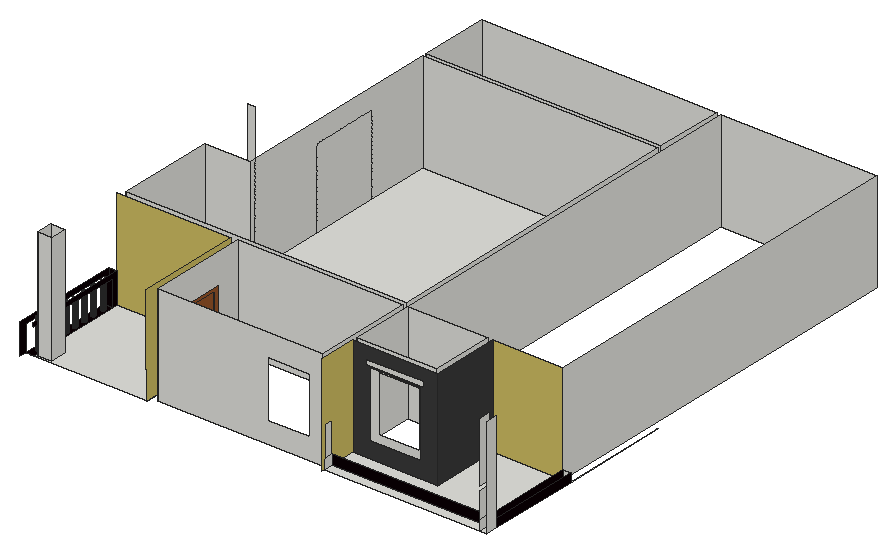
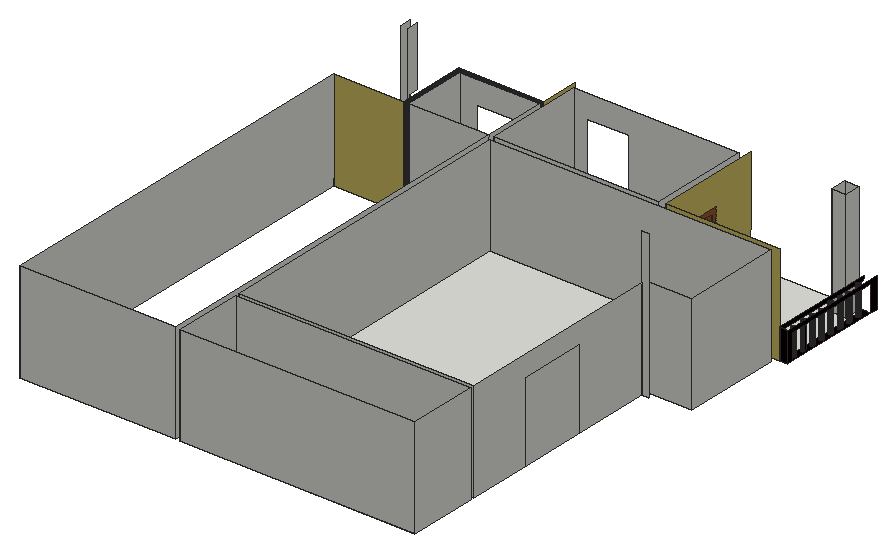
# SketchUp Ruby script. Lengths in inches.
U = 1.inch
M = Sketchup.active_model
def pt(a) = Geom::Point3d.new(a.map { |v| v * U })
def face(e, loops, mat)
  f = e.add_face(loops[0].map { |a| pt(a) })
  loops[1..].each { |l| e.add_face(l.map { |a| pt(a) }).erase! }
  f.material = f.back_material = mat if mat
  f
end
# faces: each face lists its corners as indices into pts; further lists are holes
def faces(e, pts, list, mat = nil) = list.each { |f| face(e, (f[0].is_a?(Array) ? f : [f]).map { |l| l.map { |i| pts[i] } }, mat) }
# xy, xz, yz: faces in a plane at the given z, y or x. An outline is a flat list of corners, or four numbers for a rectangle; further outlines are holes
def ring(l) = l.size == 4 ? [[l[0], l[1]], [l[2], l[1]], [l[2], l[3]], [l[0], l[3]]] : l.each_slice(2).to_a
def flat(e, list, mat, &to3) = list.each { |f| face(e, (f[0].is_a?(Array) ? f : [f]).map { |l| ring(l).map { |u, v| to3.(u, v) } }, mat) }
def xy(e, z, list, mat = nil) = flat(e, list, mat) { |x, y| [x, y, z] }
def xz(e, y, list, mat = nil) = flat(e, list, mat) { |x, z| [x, y, z] }
def yz(e, x, list, mat = nil) = flat(e, list, mat) { |y, z| [x, y, z] }
def lines(e, pts, list) = list.each { |a, b| e.add_line(pt(pts[a]), pt(pts[b])) }
# prism: a flat outline (further loops are holes) pulled along v
def prism(e, loops, v, mat = nil)
  f = face(e, loops, mat); d = Geom::Vector3d.new(v.map { |x| x * U })
  f.pushpull(f.normal.samedirection?(d) ? d.length : -d.length)
end
def box(e, o, s, mat = nil) = prism(e, [[o, [o[0] + s[0], o[1], o[2]], [o[0] + s[0], o[1] + s[1], o[2]], [o[0], o[1] + s[1], o[2]]]], [0, 0, s[2]], mat)
def at(x, y, z, deg = 0) = Geom::Transformation.translation(pt([x, y, z])) * Geom::Transformation.rotation(ORIGIN, Z_AXIS, deg.degrees)
def axes(o, x, y, z) = Geom::Transformation.new([*x, 0, *y, 0, *z, 0, *pt(o).to_a, 1])
def part(name) = M.definitions.add(name)
# library, detail: a bought-in or finely detailed component or shape, given as its bounding box
def library(name, o, s) = part(name).tap { |d| box(d.entities, o, s) }
def detail(e, o, s) = box(e.add_group.entities, o, s)
def put(e, d, t, mat = nil) = e.add_instance(d, t).tap { |i| i.material = mat if mat }
def group(e, t, mat = nil) = e.add_group.tap { |g| g.transformation = t; g.material = mat if mat }.entities
root = M.entities
M.materials.add("[Color D05]").color = [208, 191, 99]
M.materials.add("[Color E01]").color = [255, 255, 204]
M.materials.add("[Color M07]").color = [58, 58, 58]
M.materials.add("[Metal Seamed]").color = [11, 0, 4]
M.materials.add("[Wood Cherry Original]").color = [152, 86, 42]
c1 = part("Group\#1")
xy(c1.entities,0,[[0,0,6.3125,48]],"[Wood Cherry Original]")
xy(c1.entities,4.83,[[2.3125,4.83,3.9375,43.17]])
xy(c1.entities,4.83,[[0,4.83,2.3125,43.17],[3.9375,4.83,6.3125,43.17]],"[Wood Cherry Original]")
xy(c1.entities,79.17,[[2.3125,4.83,3.9375,43.17]])
xy(c1.entities,79.17,[[0,4.83,2.3125,43.17],[3.9375,4.83,6.3125,43.17]],"[Wood Cherry Original]")
xy(c1.entities,84,[[0,0,6.3125,48]],"[Wood Cherry Original]")
xz(c1.entities,0,[[0,0,6.3125,84]],"[Wood Cherry Original]")
xz(c1.entities,4.83,[[2.3125,4.83,3.9375,79.17]])
xz(c1.entities,4.83,[[0,4.83,2.3125,79.17],[3.9375,4.83,6.3125,79.17]],"[Wood Cherry Original]")
xz(c1.entities,43.17,[[2.3125,4.83,3.9375,79.17]])
xz(c1.entities,43.17,[[0,4.83,2.3125,79.17],[3.9375,4.83,6.3125,79.17]],"[Wood Cherry Original]")
xz(c1.entities,48,[[0,0,6.3125,84]],"[Wood Cherry Original]")
yz(c1.entities,0,[[[0,0,48,84],[4.83,4.83,43.17,79.17]]],"[Wood Cherry Original]")
yz(c1.entities,2.3125,[[7.68,9.76,40.37,11.76],[7.68,18.32,40.37,20.32],[7.68,27.01,40.37,29.01],[7.68,35.69,40.37,37.69],[7.68,44.38,40.37,46.38],
  [7.68,53.07,40.37,55.07],[7.68,61.76,40.37,63.76],[7.68,70.44,40.37,72.44]],"[Color E01]")
yz(c1.entities,2.3125,[[[4.83,4.83,43.17,79.17],[7.68,70.44,40.37,72.44],[7.68,61.76,40.37,63.76],[7.68,53.07,40.37,55.07],[7.68,44.38,40.37,46.38],[7.68,35.69,40.37,37.69],[7.68,27.01,40.37,29.01],[7.68,18.32,40.37,20.32],[7.68,9.76,40.37,11.76]]],"[Wood Cherry Original]")
yz(c1.entities,3.9375,[[4.83,4.83,43.17,79.17]],"[Wood Cherry Original]")
yz(c1.entities,6.3125,[[[0,0,48,84],[4.83,4.83,43.17,79.17]]],"[Wood Cherry Original]")
xy(root,288,[[[21.75,70.73,158,195.41],[24.07,73.08,41.19,92.83]],[369.3125,70.97,555.7,82.57],[555.7,70.97,564.5,84.18],[24.07,73.08,41.19,92.83],[16.88,80.51,16.29,80.625,15.75,80.89,15.29,81.28,14.95,81.78,14.75,82.35,14.7,82.95,14.82,83.55,15.08,84.09,15.47,84.55,15.97,84.89,16.54,85.09,17.14,85.13,17.74,85.02,18.28,84.76,18.74,84.36,19.08,83.86,19.28,83.29,19.32,82.69,19.21,82.1,18.95,81.55,18.55,81.1,18.05,80.76,17.49,80.56],
  [369.3125,82.57,555.7,82.57,555.7,84.18,555.3125,195.41,471.3125,195.41,471.3125,113.66,369.3125,113.66],[555.7,84.18,555.3125,195.41,564.5,195.41,564.5,84.18],[16.88,94.39,16.29,94.5,15.75,94.76,15.29,95.16,14.95,95.66,14.75,96.23,14.7,96.83,14.82,97.42,15.08,97.96,15.47,98.42,15.97,98.76,16.54,98.96,17.14,99.01,17.74,98.89,18.28,98.63,18.74,98.24,19.08,97.74,19.28,97.17,19.32,96.57,19.21,95.97,18.95,95.43,18.55,94.97,18.05,94.63,17.49,94.43],[16.88,108.26,16.29,108.375,15.75,108.64,15.29,109.03,14.95,109.53,14.75,110.1,14.7,110.7,14.82,111.3,15.08,111.84,15.47,112.3,15.97,112.64,16.54,112.84,17.14,112.88,17.74,112.77,18.28,112.51,18.74,112.11,19.08,111.61,19.28,111.04,19.32,110.44,19.21,109.85,18.95,109.3,18.55,108.85,18.05,108.51,17.49,108.31],[158,120.11,165.5625,168.11],
  [16.88,122.14,16.29,122.25,15.75,122.51,15.29,122.91,14.95,123.41,14.75,123.98,14.7,124.58,14.82,125.17,15.08,125.71,15.47,126.17,15.97,126.51,16.54,126.71,17.14,126.76,17.74,126.64,18.28,126.38,18.74,125.99,19.08,125.49,19.28,124.92,19.32,124.32,19.21,123.72,18.95,123.18,18.55,122.72,18.05,122.38,17.49,122.18],[16.88,136.01,16.29,136.125,15.75,136.39,15.29,136.78,14.95,137.28,14.75,137.85,14.7,138.45,14.82,139.05,15.08,139.59,15.47,140.05,15.97,140.39,16.54,140.59,17.14,140.63,17.74,140.52,18.28,140.26,18.74,139.86,19.08,139.36,19.28,138.79,19.32,138.19,19.21,137.6,18.95,137.05,18.55,136.6,18.05,136.26,17.49,136.06],[16.88,149.89,16.29,150,15.75,150.26,15.29,150.66,14.95,151.16,14.75,151.73,14.7,152.33,14.82,152.92,15.08,153.46,15.47,153.92,15.97,154.26,16.54,154.46,17.14,154.51,17.74,154.39,18.28,154.13,18.74,153.74,19.08,153.24,19.28,152.67,19.32,152.07,19.21,151.47,18.95,150.93,18.55,150.47,18.05,150.13,17.49,149.93],[16.88,163.76,16.29,163.875,15.75,164.14,15.29,164.53,14.95,165.03,14.75,165.6,14.7,166.2,14.82,166.8,15.08,167.34,15.47,167.8,15.97,168.14,16.54,168.34,17.14,168.38,17.74,168.27,18.28,168.01,18.74,167.61,19.08,167.11,19.28,166.54,19.32,165.94,19.21,165.35,18.95,164.8,18.55,164.35,18.05,164.01,17.49,163.81],[16.88,177.64,16.29,177.75,15.75,178.01,15.29,178.41,14.95,178.91,14.75,179.48,14.7,180.08,14.82,180.67,15.08,181.21,15.47,181.67,15.97,182.01,16.54,182.21,17.14,182.26,17.74,182.14,18.28,181.88,18.74,181.49,19.08,180.99,19.28,180.42,19.32,179.82,19.21,179.22,18.95,178.68,18.55,178.22,18.05,177.88,17.49,177.68],
  [11.6875,188.88,21.75,195.41],[564.3125,195.41,564.5,326.53],[26.75,201.41,363.3125,201.41,363.3125,578.04,81.6875,578.04,81.6875,320.85,26.75,320.85],[81.6875,582.91,363.3125,665.75]])
xy(root,288,[[[11.6875,71.13,16.3,71.13,16.54,71.21,17.14,71.26,17.74,71.14,17.77,71.13,21.75,71.13,21.75,188.88,11.6875,188.88],[16.88,163.76,16.29,163.875,15.75,164.14,15.29,164.53,14.95,165.03,14.75,165.6,14.7,166.2,14.82,166.8,15.08,167.34,15.47,167.8,15.97,168.14,16.54,168.34,17.14,168.38,17.74,168.27,18.28,168.01,18.74,167.61,19.08,167.11,19.28,166.54,19.32,165.94,19.21,165.35,18.95,164.8,18.55,164.35,18.05,164.01,17.49,163.81],[16.88,149.89,16.29,150,15.75,150.26,15.29,150.66,14.95,151.16,14.75,151.73,14.7,152.33,14.82,152.92,15.08,153.46,15.47,153.92,15.97,154.26,16.54,154.46,17.14,154.51,17.74,154.39,18.28,154.13,18.74,153.74,19.08,153.24,19.28,152.67,19.32,152.07,19.21,151.47,18.95,150.93,18.55,150.47,18.05,150.13,17.49,149.93],[16.88,136.01,16.29,136.125,15.75,136.39,15.29,136.78,14.95,137.28,14.75,137.85,14.7,138.45,14.82,139.05,15.08,139.59,15.47,140.05,15.97,140.39,16.54,140.59,17.14,140.63,17.74,140.52,18.28,140.26,18.74,139.86,19.08,139.36,19.28,138.79,19.32,138.19,19.21,137.6,18.95,137.05,18.55,136.6,18.05,136.26,17.49,136.06],[16.88,122.14,16.29,122.25,15.75,122.51,15.29,122.91,14.95,123.41,14.75,123.98,14.7,124.58,14.82,125.17,15.08,125.71,15.47,126.17,15.97,126.51,16.54,126.71,17.14,126.76,17.74,126.64,18.28,126.38,18.74,125.99,19.08,125.49,19.28,124.92,19.32,124.32,19.21,123.72,18.95,123.18,18.55,122.72,18.05,122.38,17.49,122.18],[16.88,108.26,16.29,108.375,15.75,108.64,15.29,109.03,14.95,109.53,14.75,110.1,14.7,110.7,14.82,111.3,15.08,111.84,15.47,112.3,15.97,112.64,16.54,112.84,17.14,112.88,17.74,112.77,18.28,112.51,18.74,112.11,19.08,111.61,19.28,111.04,19.32,110.44,19.21,109.85,18.95,109.3,18.55,108.85,18.05,108.51,17.49,108.31],[16.88,94.39,16.29,94.5,15.75,94.76,15.29,95.16,14.95,95.66,14.75,96.23,14.7,96.83,14.82,97.42,15.08,97.96,15.47,98.42,15.97,98.76,16.54,98.96,17.14,99.01,17.74,98.89,18.28,98.63,18.74,98.24,19.08,97.74,19.28,97.17,19.32,96.57,19.21,95.97,18.95,95.43,18.55,94.97,18.05,94.63,17.49,94.43],[16.88,80.51,16.29,80.625,15.75,80.89,15.29,81.28,14.95,81.78,14.75,82.35,14.7,82.95,14.82,83.55,15.08,84.09,15.47,84.55,15.97,84.89,16.54,85.09,17.14,85.13,17.74,85.02,18.28,84.76,18.74,84.36,19.08,83.86,19.28,83.29,19.32,82.69,19.21,82.1,18.95,81.55,18.55,81.1,18.05,80.76,17.49,80.56],[16.88,177.64,16.29,177.75,15.75,178.01,15.29,178.41,14.95,178.91,14.75,179.48,14.7,180.08,14.82,180.67,15.08,181.21,15.47,181.67,15.97,182.01,16.54,182.21,17.14,182.26,17.74,182.14,18.28,181.88,18.74,181.49,19.08,180.99,19.28,180.42,19.32,179.82,19.21,179.22,18.95,178.68,18.55,178.22,18.05,177.88,17.49,177.68]]],"[Metal Seamed]")
xz(root,73.08,[[24.07,288,41.19,420.5]])
xz(root,76.28,[[[165.5625,288,363.3125,408],[297.45,313.04,347.52,380.98]]])
xz(root,82.57,[[369.3125,288,555.7,300]],"[Metal Seamed]")
xz(root,84.18,[[555.7,288,564.5,298.1875]])
xz(root,92.83,[[24.07,288,41.19,420.5]])
xz(root,113.66,[[[369.3125,288,471.3125,408],[389.45,307.48,450.64,386.54],[384.5,386.56,384.5,393.87,454.38,393.87,454.38,386.56,450.58,386.56,450.58,386.84,390.89,386.84,390.89,386.56]]],"[Color M07]")
xz(root,119.66,[[[369.3125,288,465.3125,408],[395.02,313.04,445.08,380.98]]])
xz(root,120.11,[[158,288,165.5625,372]])
xz(root,168.11,[[158,288,165.5625,372]])
xz(root,188.88,[[11.6875,288,21.75,318.96]],"[Metal Seamed]")
xz(root,195.41,[[165.5625,288,363.3125,408],[369.3125,288,465.3125,408],[555.3125,288,564.3125,298.1875],[564.3125,288,564.5,298.1875]])
xz(root,195.41,[[21.75,288,158,408],[471.3125,288,555.3125,408]],"[Color D05]")
xz(root,195.41,[[11.6875,288,21.75,324]],"[Metal Seamed]")
xz(root,201.41,[[26.75,288,363.3125,408]])
xz(root,320.85,[[26.75,288,81.6875,408]])
xz(root,326.53,[[72.6875,288,81.6875,464.125]])
xz(root,578.04,[[81.6875,288,363.3125,408]])
xz(root,582.91,[[81.6875,288,363.3125,408]])
xz(root,664.97,[[369.3125,288,555.3125,408]])
xz(root,665.75,[[81.6875,288,363.3125,408]])
yz(root,11.6875,[[62.76,288,62.76,324,195.41,324,195.41,288,188.88,288,188.88,318.96,71.13,318.96,71.13,288]],"[Metal Seamed]")
yz(root,21.75,[[188.88,288,195.41,288,195.41,324,69.57,324,69.57,320.52,71.13,320.52,71.13,318.96,188.88,318.96]],"[Metal Seamed]")
yz(root,24.07,[[73.08,288,92.83,420.5]])
yz(root,26.75,[[201.41,288,320.85,408]])
yz(root,41.19,[[73.08,288,92.83,420.5]])
yz(root,81.6875,[[320.85,288,326.53,408],[326.53,288,419.61,288,419.61,383.34,501.8,383.34,501.8,288,578.04,288,578.04,408,326.53,408],[419.61,288,501.8,383.34],[582.91,288,665.75,408]])
yz(root,158,[[69.57,288,69.57,324,67.28,324,67.28,408,195.41,408,195.41,288,168.11,288,168.11,372,120.11,372,120.11,288]],"[Color D05]")
yz(root,165.5625,[[76.28,288,120.11,288,120.11,372,168.11,372,168.11,288,195.41,288,195.41,408,76.28,408]])
yz(root,363.3125,[[76.28,288,195.41,408],[201.41,288,578.04,408],[582.91,288,665.75,408]])
yz(root,369.3125,[[70.97,288,82.57,300],[119.66,288,195.41,408],[195.41,288,664.97,408]])
yz(root,369.3125,[[67.28,288,70.97,288,70.97,336,82.57,336,82.57,288,113.66,288,113.66,408,67.28,408]],"[Color D05]")
yz(root,465.3125,[[119.66,288,195.41,408]])
yz(root,471.3125,[[113.66,288,195.41,408]],"[Color M07]")
yz(root,555.3125,[[195.41,288,664.97,408]])
yz(root,555.7,[[70.97,288,82.57,300],[82.57,288,82.57,300,70.97,300,70.97,331.08,82.57,331.08,82.57,336,70.97,336,70.97,408,84.18,408,84.18,288]])
yz(root,564.5,[[70.97,288,84.18,408]])
yz(root,564.5,[[84.18,288,195.41,298.1875]],"[Metal Seamed]")
p = [[16.29,80.625,288],[16.88,80.51,288],[16.88,80.51,322.6875],[16.29,80.625,322.6875],[17.49,80.56,288],[17.49,80.56,322.6875],
  [15.75,80.89,288],[15.75,80.89,322.6875],[18.05,80.76,288],[18.05,80.76,322.6875],[18.55,81.1,288],[18.55,81.1,322.6875],
  [15.29,81.28,288],[15.29,81.28,322.6875],[18.95,81.55,288],[18.95,81.55,322.6875],[14.95,81.78,288],[14.95,81.78,322.6875],
  [19.21,82.1,288],[19.21,82.1,322.6875],[14.75,82.35,288],[14.75,82.35,322.6875],[19.32,82.69,288],[19.32,82.69,322.6875],
  [14.7,82.95,288],[14.7,82.95,322.6875],[19.28,83.29,288],[19.28,83.29,322.6875],[14.82,83.55,288],[14.82,83.55,322.6875],
  [19.08,83.86,288],[19.08,83.86,322.6875],[15.08,84.09,288],[15.08,84.09,322.6875],[18.74,84.36,288],[18.74,84.36,322.6875],
  [15.47,84.55,288],[15.47,84.55,322.6875],[555.3125,195.41,288],[555.7,84.18,288],[555.7,84.18,298.1875],[555.3125,195.41,298.1875],
  [18.28,84.76,288],[18.28,84.76,322.6875],[15.97,84.89,288],[15.97,84.89,322.6875],[17.74,85.02,288],[17.74,85.02,322.6875],
  [16.54,85.09,288],[16.54,85.09,322.6875],[17.14,85.13,288],[17.14,85.13,322.6875],[16.29,94.5,288],[16.88,94.39,288],
  [16.88,94.39,318.96],[16.29,94.5,318.96],[17.49,94.43,288],[17.49,94.43,318.96],[18.05,94.63,288],[18.05,94.63,318.96],
  [15.75,94.76,288],[15.75,94.76,318.96],[18.55,94.97,288],[18.55,94.97,318.96],[15.29,95.16,288],[15.29,95.16,318.96],
  [18.95,95.43,288],[18.95,95.43,318.96],[14.95,95.66,288],[14.95,95.66,318.96],[19.21,95.97,288],[19.21,95.97,318.96],
  [14.75,96.23,288],[14.75,96.23,318.96],[19.32,96.57,288],[19.32,96.57,318.96],[14.7,96.83,288],[14.7,96.83,318.96],
  [19.28,97.17,288],[19.28,97.17,318.96],[14.82,97.42,288],[14.82,97.42,318.96],[19.08,97.74,288],[19.08,97.74,318.96],
  [15.08,97.96,288],[15.08,97.96,318.96],[18.74,98.24,288],[18.74,98.24,318.96],[15.47,98.42,288],[15.47,98.42,318.96],
  [18.28,98.63,288],[18.28,98.63,318.96],[15.97,98.76,288],[15.97,98.76,318.96],[17.74,98.89,288],[17.74,98.89,318.96],
  [16.54,98.96,288],[16.54,98.96,318.96],[17.14,99.01,288],[17.14,99.01,318.96],[16.29,108.375,288],[16.88,108.26,288],
  [16.88,108.26,320.875],[16.29,108.375,320.875],[17.49,108.31,288],[17.49,108.31,320.875],[18.05,108.51,288],[18.05,108.51,320.875],
  [15.75,108.64,288],[15.75,108.64,320.875],[18.55,108.85,288],[18.55,108.85,320.875],[15.29,109.03,288],[15.29,109.03,320.875],
  [18.95,109.3,288],[18.95,109.3,320.875],[14.95,109.53,288],[14.95,109.53,320.875],[19.21,109.85,288],[19.21,109.85,320.875],
  [14.75,110.1,288],[14.75,110.1,320.875],[19.32,110.44,288],[19.32,110.44,320.875],[14.7,110.7,288],[14.7,110.7,320.875],
  [19.28,111.04,288],[19.28,111.04,320.875],[14.82,111.3,288],[14.82,111.3,320.875],[19.08,111.61,288],[19.08,111.61,320.875],
  [15.08,111.84,288],[15.08,111.84,320.875],[18.74,112.11,288],[18.74,112.11,320.875],[15.47,112.3,288],[15.47,112.3,320.875],
  [18.28,112.51,288],[18.28,112.51,320.875],[15.97,112.64,288],[15.97,112.64,320.875],[17.74,112.77,288],[17.74,112.77,320.875],
  [16.54,112.84,288],[16.54,112.84,320.875],[17.14,112.88,288],[17.14,112.88,320.875],[16.29,122.25,288],[16.88,122.14,288],
  [16.88,122.14,321.3125],[16.29,122.25,321.3125],[17.49,122.18,288],[17.49,122.18,321.3125],[18.05,122.38,288],[18.05,122.38,321.3125],
  [15.75,122.51,288],[15.75,122.51,321.3125],[18.55,122.72,288],[18.55,122.72,321.3125],[15.29,122.91,288],[15.29,122.91,321.3125],
  [18.95,123.18,288],[18.95,123.18,321.3125],[14.95,123.41,288],[14.95,123.41,321.3125],[19.21,123.72,288],[19.21,123.72,321.3125],
  [14.75,123.98,288],[14.75,123.98,321.3125],[19.32,124.32,288],[19.32,124.32,321.3125],[14.7,124.58,288],[14.7,124.58,321.3125],
  [19.28,124.92,288],[19.28,124.92,321.3125],[14.82,125.17,288],[14.82,125.17,321.3125],[19.08,125.49,288],[19.08,125.49,321.3125],
  [15.08,125.71,288],[15.08,125.71,321.3125],[18.74,125.99,288],[18.74,125.99,321.3125],[15.47,126.17,288],[15.47,126.17,321.3125],
  [18.28,126.38,288],[18.28,126.38,321.3125],[15.97,126.51,288],[15.97,126.51,321.3125],[17.74,126.64,288],[17.74,126.64,321.3125],
  [16.54,126.71,288],[16.54,126.71,321.3125],[17.14,126.76,288],[17.14,126.76,321.3125],[16.29,136.125,288],[16.88,136.01,288],
  [16.88,136.01,319],[16.29,136.125,319],[17.49,136.06,288],[17.49,136.06,319],[15.75,136.39,288],[15.75,136.39,319],
  [18.05,136.26,288],[18.05,136.26,319],[18.55,136.6,288],[18.55,136.6,319],[15.29,136.78,288],[15.29,136.78,319],
  [18.95,137.05,288],[18.95,137.05,319],[14.95,137.28,288],[14.95,137.28,319],[19.21,137.6,288],[19.21,137.6,319],
  [14.75,137.85,288],[14.75,137.85,319],[19.32,138.19,288],[19.32,138.19,319],[14.7,138.45,288],[14.7,138.45,319],
  [19.28,138.79,288],[19.28,138.79,319],[14.82,139.05,288],[14.82,139.05,319],[19.08,139.36,288],[19.08,139.36,319],
  [15.08,139.59,288],[15.08,139.59,319],[18.74,139.86,288],[18.74,139.86,319],[15.47,140.05,288],[15.47,140.05,319],
  [18.28,140.26,288],[18.28,140.26,319],[15.97,140.39,288],[15.97,140.39,319],[17.74,140.52,288],[17.74,140.52,319],
  [16.54,140.59,288],[16.54,140.59,319],[17.14,140.63,288],[17.14,140.63,319],[16.29,150,288],[16.88,149.89,288],
  [16.88,149.89,319.9375],[16.29,150,319.9375],[17.49,149.93,288],[17.49,149.93,319.9375],[18.05,150.13,288],[18.05,150.13,319.9375],
  [15.75,150.26,288],[15.75,150.26,319.9375],[18.55,150.47,288],[18.55,150.47,319.9375],[15.29,150.66,288],[15.29,150.66,319.9375],
  [18.95,150.93,288],[18.95,150.93,319.9375],[14.95,151.16,288],[14.95,151.16,319.9375],[19.21,151.47,288],[19.21,151.47,319.9375],
  [14.75,151.73,288],[14.75,151.73,319.9375],[19.32,152.07,288],[19.32,152.07,319.9375],[14.7,152.33,288],[14.7,152.33,319.9375],
  [19.28,152.67,288],[19.28,152.67,319.9375],[14.82,152.92,288],[14.82,152.92,319.9375],[19.08,153.24,288],[19.08,153.24,319.9375],
  [15.08,153.46,288],[15.08,153.46,319.9375],[18.74,153.74,288],[18.74,153.74,319.9375],[15.47,153.92,288],[15.47,153.92,319.9375],
  [18.28,154.13,288],[18.28,154.13,319.9375],[15.97,154.26,288],[15.97,154.26,319.9375],[17.74,154.39,288],[17.74,154.39,319.9375],
  [16.54,154.46,288],[16.54,154.46,319.9375],[17.14,154.51,288],[17.14,154.51,319.9375],[16.29,163.875,288],[16.88,163.76,288],
  [16.88,163.76,320.25],[16.29,163.875,320.25],[17.49,163.81,288],[17.49,163.81,320.25],[18.05,164.01,288],[18.05,164.01,320.25],
  [15.75,164.14,288],[15.75,164.14,320.25],[18.55,164.35,288],[18.55,164.35,320.25],[15.29,164.53,288],[15.29,164.53,320.25],
  [18.95,164.8,288],[18.95,164.8,320.25],[14.95,165.03,288],[14.95,165.03,320.25],[19.21,165.35,288],[19.21,165.35,320.25],
  [14.75,165.6,288],[14.75,165.6,320.25],[19.32,165.94,288],[19.32,165.94,320.25],[14.7,166.2,288],[14.7,166.2,320.25],
  [19.28,166.54,288],[19.28,166.54,320.25],[14.82,166.8,288],[14.82,166.8,320.25],[19.08,167.11,288],[19.08,167.11,320.25],
  [15.08,167.34,288],[15.08,167.34,320.25],[18.74,167.61,288],[18.74,167.61,320.25],[15.47,167.8,288],[15.47,167.8,320.25],
  [18.28,168.01,288],[18.28,168.01,320.25],[15.97,168.14,288],[15.97,168.14,320.25],[17.74,168.27,288],[17.74,168.27,320.25],
  [16.54,168.34,288],[16.54,168.34,320.25],[17.14,168.38,288],[17.14,168.38,320.25],[16.29,177.75,288],[16.88,177.64,288],
  [16.88,177.64,318.96],[16.29,177.75,318.96],[17.49,177.68,288],[17.49,177.68,318.96],[18.05,177.88,288],[18.05,177.88,318.96],
  [15.75,178.01,288],[15.75,178.01,318.96],[18.55,178.22,288],[18.55,178.22,318.96],[15.29,178.41,288],[15.29,178.41,318.96],
  [18.95,178.68,288],[18.95,178.68,318.96],[14.95,178.91,288],[14.95,178.91,318.96],[19.21,179.22,288],[19.21,179.22,318.96],
  [14.75,179.48,288],[14.75,179.48,318.96],[19.32,179.82,288],[19.32,179.82,318.96],[14.7,180.08,288],[14.7,180.08,318.96],
  [19.28,180.42,288],[19.28,180.42,318.96],[14.82,180.67,288],[14.82,180.67,318.96],[19.08,180.99,288],[19.08,180.99,318.96],
  [15.08,181.21,288],[15.08,181.21,318.96],[18.74,181.49,288],[18.74,181.49,318.96],[15.47,181.67,288],[15.47,181.67,318.96],
  [18.28,181.88,288],[18.28,181.88,318.96],[15.97,182.01,288],[15.97,182.01,318.96],[17.74,182.14,288],[17.74,182.14,318.96],
  [16.54,182.21,288],[16.54,182.21,318.96],[17.14,182.26,288],[17.14,182.26,318.96],[26.75,320.85,288],[26.75,326.53,288]]
faces(root,p,[[0,1,2,3],[1,4,5,2],[6,0,3,7],[4,8,9,5],[8,10,11,9],[12,6,7,13],[10,14,15,11],[16,12,13,17],
  [14,18,19,15],[20,16,17,21],[18,22,23,19],[24,20,21,25],[22,26,27,23],[28,24,25,29],[26,30,31,27],[32,28,29,33],
  [30,34,35,31],[36,32,33,37],[38,39,40,41],[34,42,43,35],[44,36,37,45],[42,46,47,43],[48,44,45,49],[46,50,51,47],
  [50,48,49,51],[52,53,54,55],[53,56,57,54],[56,58,59,57],[60,52,55,61],[58,62,63,59],[64,60,61,65],[62,66,67,63],
  [68,64,65,69],[66,70,71,67],[72,68,69,73],[70,74,75,71],[76,72,73,77],[74,78,79,75],[80,76,77,81],[78,82,83,79],
  [84,80,81,85],[82,86,87,83],[88,84,85,89],[86,90,91,87],[92,88,89,93],[90,94,95,91],[96,92,93,97],[94,98,99,95],
  [98,96,97,99],[100,101,102,103],[101,104,105,102],[104,106,107,105],[108,100,103,109],[106,110,111,107],[112,108,109,113],[110,114,115,111],
  [116,112,113,117],[114,118,119,115],[120,116,117,121],[118,122,123,119],[124,120,121,125],[122,126,127,123],[128,124,125,129],[126,130,131,127],
  [132,128,129,133],[130,134,135,131],[136,132,133,137],[134,138,139,135],[140,136,137,141],[138,142,143,139],[144,140,141,145],[146,144,145,147],
  [142,146,147,143],[148,149,150,151],[149,152,153,150],[152,154,155,153],[156,148,151,157],[154,158,159,155],[160,156,157,161],[158,162,163,159],
  [164,160,161,165],[162,166,167,163],[168,164,165,169],[166,170,171,167],[172,168,169,173],[170,174,175,171],[176,172,173,177],[174,178,179,175],
  [180,176,177,181],[178,182,183,179],[184,180,181,185],[182,186,187,183],[188,184,185,189],[186,190,191,187],[192,188,189,193],[190,194,195,191],
  [194,192,193,195],[196,197,198,199],[197,200,201,198],[202,196,199,203],[200,204,205,201],[204,206,207,205],[208,202,203,209],[206,210,211,207],
  [212,208,209,213],[210,214,215,211],[216,212,213,217],[214,218,219,215],[220,216,217,221],[218,222,223,219],[224,220,221,225],[222,226,227,223],
  [228,224,225,229],[226,230,231,227],[232,228,229,233],[230,234,235,231],[236,232,233,237],[234,238,239,235],[240,236,237,241],[238,242,243,239],
  [242,240,241,243],[244,245,246,247],[245,248,249,246],[248,250,251,249],[252,244,247,253],[250,254,255,251],[256,252,253,257],[254,258,259,255],
  [260,256,257,261],[258,262,263,259],[264,260,261,265],[262,266,267,263],[268,264,265,269],[266,270,271,267],[272,268,269,273],[270,274,275,271],
  [276,272,273,277],[274,278,279,275],[280,276,277,281],[278,282,283,279],[284,280,281,285],[282,286,287,283],[288,284,285,289],[286,290,291,287],
  [290,288,289,291],[292,293,294,295],[293,296,297,294],[296,298,299,297],[300,292,295,301],[298,302,303,299],[304,300,301,305],[302,306,307,303],
  [308,304,305,309],[306,310,311,307],[312,308,309,313],[310,314,315,311],[316,312,313,317],[314,318,319,315],[320,316,317,321],[318,322,323,319],
  [324,320,321,325],[322,326,327,323],[328,324,325,329],[326,330,331,327],[332,328,329,333],[330,334,335,331],[336,332,333,337],[338,336,337,339],
  [334,338,339,335],[340,341,342,343],[341,344,345,342],[344,346,347,345],[348,340,343,349],[346,350,351,347],[352,348,349,353],[350,354,355,351],
  [356,352,353,357],[354,358,359,355],[360,356,357,361],[358,362,363,359],[364,360,361,365],[362,366,367,363],[368,364,365,369],[366,370,371,367],
  [372,368,369,373],[370,374,375,371],[376,372,373,377],[374,378,379,375],[380,376,377,381],[378,382,383,379],[384,380,381,385],[382,386,387,383],
  [386,384,385,387]],"[Metal Seamed]")
lines(root,p,[[388,389]])
put(root,c1,at(158,120.11,288))
